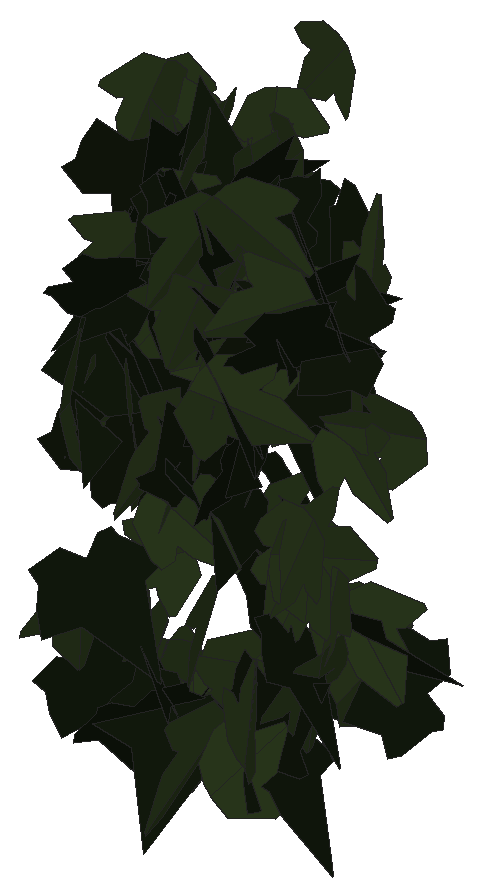
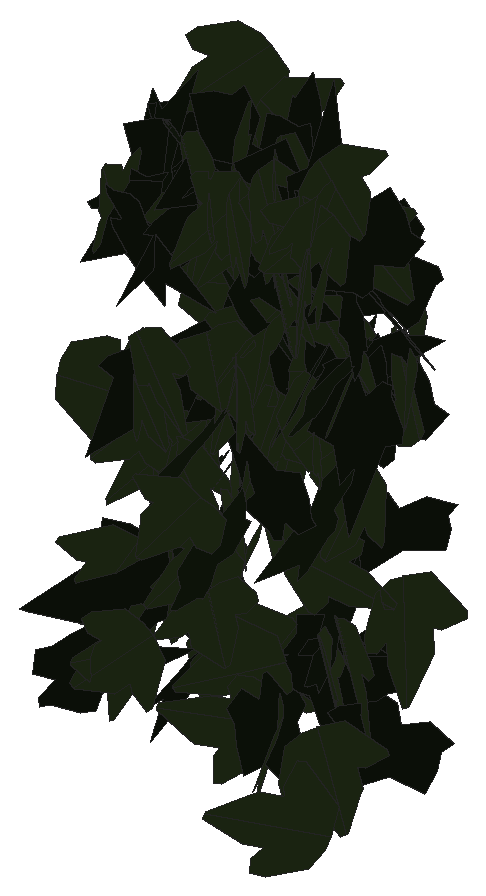
# SketchUp Ruby script. Lengths in inches.
U = 1.inch
M = Sketchup.active_model
def pt(a) = Geom::Point3d.new(a.map { |v| v * U })
def face(e, loops, mat)
  f = e.add_face(loops[0].map { |a| pt(a) })
  loops[1..].each { |l| e.add_face(l.map { |a| pt(a) }).erase! }
  f.material = f.back_material = mat if mat
  f
end
# faces: each face lists its corners as indices into pts; further lists are holes
def faces(e, pts, list, mat = nil) = list.each { |f| face(e, (f[0].is_a?(Array) ? f : [f]).map { |l| l.map { |i| pts[i] } }, mat) }
# xy, xz, yz: faces in a plane at the given z, y or x. An outline is a flat list of corners, or four numbers for a rectangle; further outlines are holes
def ring(l) = l.size == 4 ? [[l[0], l[1]], [l[2], l[1]], [l[2], l[3]], [l[0], l[3]]] : l.each_slice(2).to_a
def flat(e, list, mat, &to3) = list.each { |f| face(e, (f[0].is_a?(Array) ? f : [f]).map { |l| ring(l).map { |u, v| to3.(u, v) } }, mat) }
def xy(e, z, list, mat = nil) = flat(e, list, mat) { |x, y| [x, y, z] }
def xz(e, y, list, mat = nil) = flat(e, list, mat) { |x, z| [x, y, z] }
def yz(e, x, list, mat = nil) = flat(e, list, mat) { |y, z| [x, y, z] }
def lines(e, pts, list) = list.each { |a, b| e.add_line(pt(pts[a]), pt(pts[b])) }
# prism: a flat outline (further loops are holes) pulled along v
def prism(e, loops, v, mat = nil)
  f = face(e, loops, mat); d = Geom::Vector3d.new(v.map { |x| x * U })
  f.pushpull(f.normal.samedirection?(d) ? d.length : -d.length)
end
def box(e, o, s, mat = nil) = prism(e, [[o, [o[0] + s[0], o[1], o[2]], [o[0] + s[0], o[1] + s[1], o[2]], [o[0], o[1] + s[1], o[2]]]], [0, 0, s[2]], mat)
def at(x, y, z, deg = 0) = Geom::Transformation.translation(pt([x, y, z])) * Geom::Transformation.rotation(ORIGIN, Z_AXIS, deg.degrees)
def axes(o, x, y, z) = Geom::Transformation.new([*x, 0, *y, 0, *z, 0, *pt(o).to_a, 1])
def part(name) = M.definitions.add(name)
# library, detail: a bought-in or finely detailed component or shape, given as its bounding box
def library(name, o, s) = part(name).tap { |d| box(d.entities, o, s) }
def detail(e, o, s) = box(e.add_group.entities, o, s)
def put(e, d, t, mat = nil) = e.add_instance(d, t).tap { |i| i.material = mat if mat }
def group(e, t, mat = nil) = e.add_group.tap { |g| g.transformation = t; g.material = mat if mat }.entities
root = M.entities
M.materials.add("efeu1").color = [18, 25, 13]
M.materials.add("efeu2").color = [43, 57, 29]
c1 = part("ivyleaf_10")
p = [[0,0.5,-0.03],[-0.0625,2.02,-0.43],[-0.19,2.01,-0.46],[-0.54,1.05,-0.29],[-0.52,0.625,-0.18],[-0.83,0.76,-0.28],
  [-1.16,0.64,-0.33],[-1.15,0.33,-0.24],[-0.77,-0.39,0.02],[-0.3,-0.51,0.16],[0.04,-0.48,0.23],[-0.02,2.01,-0.4375],
  [-0.06,2.01,-0.43],[0.04,-0.49,0.23],[0.67,-0.49,0.14],[1.38,0.36,-0.2],[1.375,0.51,-0.24],[0.81,0.65,-0.19],
  [0.62,0.59,-0.15],[0.6,1.09,-0.28],[0.5,1.23,-0.31]]
faces(c1.entities,p,[[0,1,2,3,4,5,6,7,8,9,10],[11,12,0,13,14,15,16,17,18,19,20]],"efeu2")
c2 = part("ivyleaf_9")
p = [[1.54,2.16,1.25],[1.36,2.04,1.19],[-0.21,0.99,0.68],[-0.71,1.11,0.82],[-0.85,0.86,0.67],[-0.8,0.17,0.21],
  [-0.9,-0.01,0.1],[-0.67,-0.16,-0.02],[-0.08,-0.08,-0.05],[-0.03,-0.6,-0.4],[0.65,-0.88,-0.66],[0.83,-0.6,-0.49],
  [1.29,-0.42,-0.43],[1.8125,-0.07,-0.26],[1.21,0.44,0.15]]
faces(c2.entities,p,[[0,1,2,3,4,5,6,7,8,9,10,11,12,13,14]],"efeu1")
put(root,c1,axes([530.92,134.8125,174.84],[-0.19592,-0.8263,-0.09777],[0.03517,0.09213,-0.84912],[0.83133,-0.19864,0.01288]))
put(root,c1,axes([530.8,137.07,182.33],[-0.34578,0.60475,-0.1129],[0.00149,-0.12869,-0.69388],[-0.61519,-0.34022,0.06178]))
put(root,c2,axes([530.49,135.57,172.97],[-0.03225,-0.22787,-0.72539],[0.24551,0.68403,-0.2258],[0.71961,-0.24359,0.04452]))
put(root,c1,axes([530.93,136.81,183.76],[-0.21616,-0.60242,0.36221],[0.06033,-0.39345,-0.61837],[0.70033,-0.15204,0.16507]))
put(root,c1,axes([531.1,136.78,172.87],[-0.47373,-0.52814,0.19177],[-0.12666,-0.14401,-0.70948],[0.54742,-0.49037,0.0018]))
put(root,c1,axes([530.84,137.375,183.43],[0.00401,0.699,-0.0965],[-0.00277,-0.09649,-0.69901],[-0.70562,0.00436,0.0022]))
put(root,c1,axes([531.17,141.23,182.34],[0.54265,-0.19104,-0.4391],[-0.36577,0.26296,-0.56643],[0.30906,0.64663,0.10062]))
put(root,c1,axes([530.8,139.3125,181.07],[0.50318,-0.47093,0.13603],[0.20407,0.02401,-0.67175],[0.44568,0.52069,0.15401]))
put(root,c1,axes([530.88,138.6875,181.49],[-0.00418,0.69932,-0.06517],[0.00237,-0.06516,-0.69933],[-0.70235,-0.00438,-0.00197]))
put(root,c1,axes([531.07,137.29,182.21],[0.41222,-0.492,-0.30715],[-0.01427,0.3681,-0.60879],[0.57983,0.35884,0.20338]))
put(root,c2,axes([531.17,135.59,178.91],[0.54862,0.17349,-0.49669],[-0.48901,-0.09657,-0.57387],[-0.19408,0.73373,0.04191]))
put(root,c1,axes([531.05,139.83,181.88],[0.34488,0.60263,-0.13044],[-0.10314,-0.09097,-0.69297],[-0.6079,0.35733,0.04357]))
put(root,c1,axes([530.84,137.27,183.05],[-0.53243,-0.11728,-0.45636],[0.46832,-0.05584,-0.53203],[0.05192,-0.69902,0.11907]))
put(root,c1,axes([531.125,137.25,182.26],[-0.41909,0.55041,-0.16861],[-0.01192,-0.21681,-0.67814],[-0.57554,-0.3963,0.13682]))
put(root,c2,axes([530.71,136.01,181.91],[-0.09729,-0.01093,0.76292],[0.76291,-0.0131,0.0971],[0.01161,0.76899,0.01249]))
put(root,c1,axes([530.84,137.6,171.8],[-0.13787,-0.247,0.79868],[0.35271,0.71671,0.28254],[-0.75795,0.37845,-0.0138]))
put(root,c1,axes([531.63,133.63,179.07],[-0.16377,0.22479,0.89507],[-0.63854,0.62872,-0.27473],[-0.66629,-0.65778,0.04329]))
put(root,c1,axes([531.1,134.48,178.15],[0.26185,-0.71309,-0.12686],[0.04397,-0.11899,0.75965],[-0.72295,-0.26552,0.00025]))
put(root,c1,axes([531.4,135.74,174.37],[0.56044,-0.44465,-0.32134],[-0.19833,0.26408,-0.71133],[0.5115,0.58959,0.07627]))
put(root,c1,axes([531.18,135.72,177.43],[-0.74972,0.24636,-0.21773],[0.20616,-0.07006,-0.78916],[-0.25611,-0.77755,0.00212]))
put(root,c1,axes([531.76,135.16,181.71],[-0.39552,-0.42422,0.48369],[-0.3164,-0.36611,-0.57983],[0.56019,-0.50631,0.01401]))
put(root,c2,axes([531.04,136.64,177.33],[0.62812,-0.5273,-0.05641],[-0.03686,0.04382,-0.82005],[0.52902,0.62912,0.00984]))
put(root,c2,axes([531.03,136.02,181.04],[-0.05095,-0.02497,-0.76011],[0.75951,-0.04099,-0.04956],[-0.03925,-0.76071,0.02762]))
put(root,c2,axes([531.93,135.21,181.12],[-0.76866,0.26052,-0.00953],[0.00902,-0.00307,-0.81161],[-0.26054,-0.76871,0.00001]))
put(root,c2,axes([531.25,134.37,181.06],[0.59812,0.33004,0.3442],[0.30367,0.16211,-0.68312],[-0.36768,0.67078,-0.00427]))
put(root,c2,axes([531.59,135.1,179.38],[-0.32525,-0.70375,0.01057],[0.00472,-0.01383,-0.77521],[0.70381,-0.32513,0.01008]))
put(root,c1,axes([532.12,135.7,175.56],[0.31089,0.04691,-0.65176],[-0.64669,-0.08147,-0.31433],[-0.09376,0.7175,0.00692]))
put(root,c1,axes([531.82,135.74,173.92],[0.40371,-0.61922,-0.1852],[-0.10233,0.15438,-0.7392],[0.63817,0.41647,-0.00136]))
put(root,c2,axes([531.375,136.12,179.4],[0.22527,-0.71155,0.33589],[0.15397,-0.30277,-0.74464],[0.77163,0.26814,0.05052]))
put(root,c1,axes([532.06,135.42,180.14],[0.63234,-0.19799,-0.38587],[-0.37241,0.10175,-0.6625],[0.22227,0.73375,-0.01225]))
put(root,c2,axes([531.77,135.96,182.35],[0.12709,0.40881,0.63775],[-0.25597,-0.58545,0.4263],[0.71297,-0.28306,0.03937]))
put(root,c1,axes([531.98,137.16,183.28],[0.12019,-0.70701,0.0361],[-0.00248,-0.03704,-0.71711],[0.70793,0.11991,-0.00864]))
put(root,c1,axes([531.85,135.07,179.03],[-0.26711,0.68467,-0.33979],[0.12361,-0.31651,-0.73493],[-0.75429,-0.29432,-0.00011]))
put(root,c2,axes([531.71,134.0625,175.97],[-0.0097,-0.53903,-0.59916],[0.14398,0.5884,-0.53169],[0.79298,-0.11343,0.08921]))
put(root,c1,axes([532.34,135.55,177.88],[-0.3205,-0.23206,-0.65993],[-0.40562,-0.52976,0.38328],[-0.56994,0.50752,0.09832]))
put(root,c2,axes([531.62,134.3,177.67],[-0.1215,0.00874,0.81576],[0.79755,-0.17226,0.12063],[0.17165,0.80657,0.01692]))
put(root,c1,axes([532.26,135.26,177.72],[0.16697,-0.65108,-0.24893],[-0.04432,0.24554,-0.67193],[0.69563,0.17192,0.01694]))
put(root,c1,axes([532.375,136.5625,182.39],[0.45782,-0.53279,-0.20144],[-0.13274,0.15153,-0.70247],[0.55392,0.47667,-0.00184]))
put(root,c2,axes([532.43,134.4,173.32],[0.25351,0.74846,-0.2114],[-0.06839,-0.20003,-0.79022],[-0.77473,0.26257,0.00059]))
put(root,c2,axes([531.86,135.0625,178.55],[-0.19418,0.04581,0.74962],[0.60086,-0.45503,0.18345],[0.45056,0.62657,0.07841]))
put(root,c1,axes([532.7,136.11,182.23],[-0.323,-0.26817,0.6358],[-0.39448,-0.50422,-0.41308],[0.56617,-0.50432,0.07491]))
put(root,c1,axes([532.39,136.16,183.3],[0.19541,-0.6819,-0.25984],[-0.01407,0.26543,-0.70713],[0.72959,0.18775,0.05596]))
put(root,c2,axes([532.62,136.47,173.06],[-0.36985,0.55326,-0.3839],[0.20615,-0.32395,-0.66546],[-0.64108,-0.42336,0.00749]))
put(root,c1,axes([532.375,136.47,172.65],[-0.35173,0.64738,-0.21219],[0.1062,-0.18378,-0.73674],[-0.67294,-0.36737,-0.00536]))
put(root,c2,axes([532.24,136.43,176.74],[-0.27261,0.2541,0.67706],[0.49979,-0.45676,0.37265],[0.52267,0.56929,-0.00321]))
put(root,c2,axes([532.36,135.7,182.66],[0.28666,-0.62756,-0.34449],[-0.13402,0.31747,-0.68987],[0.70323,0.31632,0.00895]))
put(root,c2,axes([532.1,135.14,174.06],[0.44411,-0.13885,-0.6961],[0.65846,-0.22608,0.46519],[-0.2651,-0.79416,-0.01072]))
put(root,c2,axes([532.43,135.72,182.52],[0.01568,-0.56773,-0.52209],[-0.01541,0.52186,-0.56794],[0.77114,0.02197,-0.00074]))
put(root,c2,axes([533.06,135.93,182.3],[-0.79601,-0.10524,0.07959],[0.07911,0.00886,0.80293],[-0.1056,0.79993,0.00158]))
put(root,c1,axes([532.69,137.08,182.58],[0.2606,-0.65105,0.14646],[0.1525,-0.09497,-0.69351],[0.64967,0.28345,0.10404]))
put(root,c1,axes([532.61,135.95,180.76],[0.68747,-0.39553,0.27155],[0.23727,-0.13212,-0.79313],[0.417,0.72726,0.0036]))
put(root,c1,axes([532.8125,137.6,175.41],[0.36108,0.61203,-0.161],[-0.09946,-0.12818,-0.71032],[-0.62498,0.37399,0.02003]))
put(root,c2,axes([533.09,135.22,177.93],[0.14685,-0.82199,0.35173],[-0.04027,0.35,0.83477],[-0.89318,-0.15093,0.0202]))
put(root,c2,axes([532.38,138.02,176.52],[0.28891,-0.58933,0.41729],[0.26811,-0.32978,-0.65137],[0.6705,0.38581,0.08065]))
put(root,c1,axes([532.83,134.9375,178.5625],[0.08804,-0.37842,0.85664],[0.24966,-0.81979,-0.38781],[0.90261,0.26367,0.02371]))
put(root,c1,axes([532.91,136.93,182.58],[0.10694,0.24991,0.66756],[-0.04941,0.676,-0.24515],[-0.71109,-0.00939,0.11742]))
put(root,c2,axes([532.95,135.06,173.22],[-0.46331,-0.71241,-0.10635],[0.05627,0.09027,-0.84981],[0.7181,-0.46671,-0.00202]))
put(root,c1,axes([532.61,138.39,177.63],[0.50346,0.22872,0.47666],[0.40646,0.25347,-0.55094],[-0.3381,0.64531,0.04746]))
put(root,c1,axes([533.05,135,177.4],[0.00317,-0.65593,-0.41451],[0.07918,0.41262,-0.65234],[0.77187,-0.03964,0.06862]))
put(root,c1,axes([533.11,135.5,177.94],[-0.06259,-0.54008,-0.55234],[0.04985,0.55017,-0.54361],[0.7709,-0.07942,-0.00969]))
put(root,c1,axes([532.98,136.64,176.17],[0.21437,-0.45477,-0.58097],[0.23911,-0.52952,0.50272],[-0.69797,-0.32107,-0.00621]))
put(root,c1,axes([533.44,135.3,181.5],[-0.50631,-0.48638,-0.37022],[-0.23565,-0.28825,0.70097],[-0.564,0.55707,0.03947]))
put(root,c1,axes([533.1,135.95,179.83],[0.08431,0.54944,0.5275],[0.10267,0.51768,-0.55563],[-0.75472,0.1318,-0.01666]))
put(root,c2,axes([533.1,135.6875,180.08],[0.07368,0.61367,0.4652],[-0.09956,-0.45581,0.61705],[0.7636,-0.11864,0.03557]))
put(root,c1,axes([533.37,136.04,179.06],[-0.07849,-0.59345,-0.48082],[0.05655,0.47751,-0.5986],[0.76169,-0.0966,-0.0051]))
put(root,c1,axes([533.23,136.92,176.1],[-0.17232,-0.34701,-0.67658],[0.32756,0.59219,-0.38715],[0.68621,-0.36982,0.01491]))
put(root,c1,axes([533.67,134.5,181.54],[-0.55634,-0.48954,0.26481],[-0.19791,-0.17595,-0.74105],[0.52019,-0.59049,0.00127]))
put(root,c1,axes([532.96,136.01,173.48],[0.18103,0.13128,0.73059],[0.51774,0.51655,-0.22111],[-0.53192,0.54745,0.03343]))
put(root,c2,axes([533.17,134.71,181.27],[0.75465,0.09488,-0.06699],[-0.06764,0.00101,-0.76053],[-0.09442,0.75761,0.0094]))
put(root,c1,axes([533.97,135.65,173.51],[-0.58116,-0.26975,0.60397],[-0.54847,-0.25289,-0.64071],[0.36975,-0.79911,-0.00112]))
put(root,c1,axes([533.72,136.95,183.22],[0.39434,-0.29593,-0.5332],[-0.33987,0.42056,-0.48477],[0.50633,0.51277,0.08987]))
put(root,c1,axes([533.43,135.03,172.84],[0.15464,-0.56166,0.72735],[0.14854,-0.7126,-0.58185],[0.90688,0.21249,-0.02872]))
put(root,c2,axes([532.875,135.31,182.32],[0.72354,-0.13953,0.39052],[0.38965,-0.04003,-0.73624],[0.14192,0.82123,0.03046]))
put(root,c1,axes([533.05,136.09,172.38],[0.15517,0.12249,-0.80697],[0.66206,0.46153,0.19736],[0.47737,-0.6799,-0.01141]))
put(root,c1,axes([533.7,134.6875,182.95],[-0.14771,-0.68776,0.50868],[-0.0904,-0.50077,-0.70332],[0.85065,-0.17264,0.01359]))
put(root,c1,axes([533.24,136.22,182.87],[0.19775,-0.19404,0.71795],[0.45517,-0.55593,-0.27562],[0.58815,0.49548,-0.02808]))
put(root,c2,axes([533.15,137.69,178.11],[0.27904,-0.71441,0.17284],[0.08645,-0.1517,-0.76657],[0.72992,0.29108,0.02471]))
put(root,c2,axes([533.08,134.89,182.55],[0.17379,-0.22307,0.73051],[0.40252,-0.60996,-0.28202],[0.64914,0.43795,-0.0207]))
put(root,c1,axes([533.08,134.39,177.4],[0.34167,0.1764,0.68235],[0.62031,0.2847,-0.38421],[-0.33456,0.70801,-0.01551]))
put(root,c2,axes([533.63,134.68,177.9],[0.54873,0.18542,0.54182],[-0.51011,-0.18278,0.57917],[0.26027,-0.74918,-0.0072]))
put(root,c2,axes([533.5625,135.68,182.95],[0.27074,0.4641,0.56482],[0.26469,0.49921,-0.53707],[-0.68143,0.3783,0.01579]))
put(root,c1,axes([533.6875,134.85,175.76],[0.31306,-0.65939,0.28538],[0.15154,-0.2437,-0.72931],[0.70234,0.34649,0.03015]))
put(root,c2,axes([533.67,134.58,178.75],[-0.09642,0.68746,-0.48853],[-0.12936,0.47384,0.69231],[0.83338,0.15309,0.05094]))
put(root,c1,axes([534.27,135.74,180.21],[0.16584,0.08347,-0.82387],[-0.70703,-0.42315,-0.18519],[-0.4311,0.7261,-0.01322]))
put(root,c2,axes([533.57,135.78,177.29],[0.01318,-0.6663,0.50954],[0.03933,-0.50855,-0.66602],[0.83788,0.03435,0.02324]))
put(root,c1,axes([533.82,135.58,181.74],[-0.22728,-0.56293,-0.48951],[0.18668,0.45253,-0.60707],[0.72226,-0.29411,0.00287]))
put(root,c1,axes([533.42,135.49,180.85],[-0.39834,-0.1554,0.62294],[0.61976,0.09837,0.42084],[-0.16766,0.73284,0.07561]))
put(root,c2,axes([534.13,134.66,178.36],[-0.21523,0.40011,-0.72287],[-0.43968,0.57697,0.45026],[0.69951,0.48576,0.0606]))
put(root,c2,axes([533.75,136.74,182.29],[0.31539,-0.46545,-0.56839],[-0.17936,0.55105,-0.55077],[0.71242,0.34479,0.11296]))
put(root,c1,axes([533.88,134.52,180.01],[0.58671,-0.49198,0.27184],[0.21448,-0.16726,-0.76563],[0.51956,0.62462,0.00909]))
put(root,c2,axes([534.1875,135.73,175.27],[0.22285,-0.69647,0.25184],[-0.03381,0.25316,0.73002],[-0.73984,-0.22136,0.0425]))
put(root,c1,axes([534.51,137.4,179.125],[0.29985,-0.10603,-0.82326],[-0.55575,0.62454,-0.28285],[0.61656,0.61451,0.14543]))
put(root,c2,axes([534.52,135.11,180.36],[-0.70669,0.43793,-0.15557],[0.13282,-0.08101,-0.83138],[-0.44536,-0.71906,-0.00108]))
put(root,c2,axes([534.95,137.14,181.61],[-0.34965,-0.06598,-0.81149],[-0.80047,-0.13349,0.35575],[-0.14875,0.87347,-0.00692]))
put(root,c2,axes([534.78,135.92,182.73],[-0.6837,0.35652,0.01757],[-0.01695,0.0055,-0.77107],[-0.35655,-0.6839,0.00296]))
put(root,c2,axes([534.13,137.04,179.27],[-0.00413,-0.36844,-0.6807],[0.05702,0.67872,-0.36771],[0.77192,-0.05211,0.02352]))
put(root,c1,axes([534.15,137.95,174.29],[-0.5428,0.05706,-0.5071],[0.5046,-0.05025,-0.54579],[-0.07601,-0.74112,-0.00204]))
put(root,c1,axes([534.54,135.77,181.54],[0.59592,0.4652,-0.14589],[-0.11444,-0.0905,-0.75599],[-0.47392,0.6068,-0.0009]))
put(root,c2,axes([534.02,134.76,180.01],[0.28054,-0.58906,0.69287],[0.27017,-0.63837,-0.65211],[0.86837,0.38892,-0.02095]))
put(root,c1,axes([534.31,134.49,172.57],[0.57608,-0.06691,-0.43727],[0.4423,0.09879,0.56759],[0.00719,-0.71646,0.1191]))
put(root,c1,axes([534.95,134.09,173.64],[-0.0446,0.3922,-0.6869],[-0.18265,0.66429,0.39115],[0.76961,0.18038,0.05302]))
put(root,c2,axes([535.13,135.63,181.3125],[-0.0248,0.13987,-0.83926],[-0.19619,-0.81794,-0.13052],[-0.82791,0.18963,0.05607]))
put(root,c2,axes([534.64,135.49,172.82],[0.28026,-0.66014,-0.30936],[-0.09504,0.29552,-0.7167],[0.72281,0.29482,0.02571]))
put(root,c2,axes([535.08,135.29,180.82],[0.12021,-0.56989,0.53563],[0.03626,0.5454,0.57215],[-0.78126,-0.06237,0.10897]))
put(root,c2,axes([534.49,135.17,173.26],[-0.14892,0.12526,0.76329],[0.54982,-0.5296,0.19418],[0.54406,0.56949,0.01269]))
put(root,c1,axes([534.9,136.96,173.49],[0.04169,0.2036,-0.79346],[0.20559,0.76646,0.20747],[0.79295,-0.20942,-0.01208]))
put(root,c1,axes([534.6,134.34,183.64],[-0.54952,-0.12956,-0.59148],[0.58533,0.09081,-0.56369],[0.155,-0.80223,0.03172]))
put(root,c1,axes([534.54,133.86,180.26],[-0.35345,-0.24827,-0.7794],[0.71573,0.3172,-0.42562],[0.39603,-0.79484,0.0736]))
put(root,c1,axes([535.57,134.65,182.05],[-0.27258,-0.19184,0.73741],[-0.56136,-0.47901,-0.33213],[0.51523,-0.6234,0.02827]))
put(root,c1,axes([535.18,135.38,176.375],[0.77668,-0.21632,-0.2135],[-0.20694,0.05272,-0.80623],[0.2226,0.80376,-0.00457]))
put(root,c1,axes([534.66,137.14,178],[0.51802,0.05372,0.52739],[0.51219,0.13943,-0.5173],[-0.1367,0.72598,0.06032]))
put(root,c2,axes([535.65,137.98,173.17],[-0.33959,-0.20304,0.67929],[-0.59233,-0.33266,-0.39556],[0.38962,-0.68271,-0.00928]))
put(root,c1,axes([535.8125,137.26,178.44],[0.06338,0.08455,-0.74239],[-0.74682,0.03041,-0.0603],[0.02331,0.74447,0.08678]))
put(root,c1,axes([535.1875,135.21,176.82],[0.00011,0.324,0.86638],[-0.03275,0.86584,-0.3238],[-0.9244,-0.03064,0.01158]))
put(root,c2,axes([535.08,135.05,181.52],[0.41336,0.56215,0.56458],[0.34914,0.44391,-0.69762],[-0.71615,0.54089,-0.01424]))
put(root,c1,axes([535.52,134.89,177.44],[0.74736,-0.32915,-0.18532],[-0.16942,0.07511,-0.81663],[0.33762,0.76632,0.00045]))
put(root,c1,axes([535.56,135.3,174.76],[-0.02997,-0.89458,-0.09511],[0.00353,0.09505,-0.89508],[0.89961,-0.03017,0.00034]))
put(root,c2,axes([534.9,136.72,174.61],[0.63996,-0.05397,0.40628],[0.408,0.01244,-0.64102],[0.03887,0.75793,0.03945]))
put(root,c1,axes([535.61,136.58,181.57],[-0.06767,0.56097,-0.48379],[-0.05638,0.48049,0.56504],[0.73862,0.08807,-0.00119]))
put(root,c1,axes([535.44,135.78,176.01],[0.70918,-0.32315,0.10312],[0.09526,-0.03962,-0.77932],[0.32555,0.71554,0.00341]))
put(root,c2,axes([536.01,135.9375,181.02],[-0.32378,-0.63697,-0.36216],[-0.12763,-0.34086,0.71362],[-0.72152,0.34614,0.03628]))
put(root,c2,axes([535.24,135.01,175.37],[0.40638,-0.67778,-0.04257],[-0.02392,0.0353,-0.79027],[0.6787,0.40708,-0.00236]))
put(root,c1,axes([535.29,136.64,175.07],[0.49832,0.52107,0.39712],[0.28026,0.28144,-0.72096],[-0.59217,0.57168,-0.00703]))
put(root,c2,axes([535.34,134.11,181.41],[0.51886,0.45925,0.48026],[0.36703,0.30987,-0.69285],[-0.55393,0.63549,-0.00923]))
put(root,c2,axes([535.89,135.3125,181.5],[0.26789,-0.52039,0.52861],[-0.18266,0.49844,0.58326],[-0.71893,-0.32054,0.04878]))
